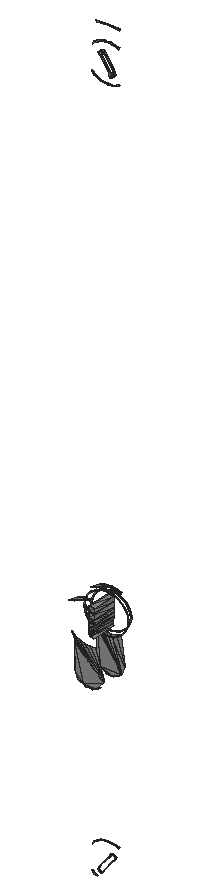
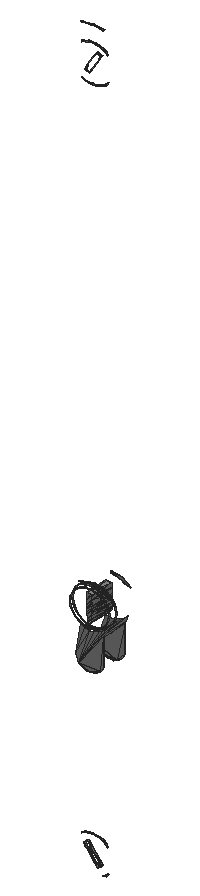
# SketchUp Ruby script. Lengths in inches.
U = 1.inch
M = Sketchup.active_model
def pt(a) = Geom::Point3d.new(a.map { |v| v * U })
def face(e, loops, mat)
  f = e.add_face(loops[0].map { |a| pt(a) })
  loops[1..].each { |l| e.add_face(l.map { |a| pt(a) }).erase! }
  f.material = f.back_material = mat if mat
  f
end
# faces: each face lists its corners as indices into pts; further lists are holes
def faces(e, pts, list, mat = nil) = list.each { |f| face(e, (f[0].is_a?(Array) ? f : [f]).map { |l| l.map { |i| pts[i] } }, mat) }
# xy, xz, yz: faces in a plane at the given z, y or x. An outline is a flat list of corners, or four numbers for a rectangle; further outlines are holes
def ring(l) = l.size == 4 ? [[l[0], l[1]], [l[2], l[1]], [l[2], l[3]], [l[0], l[3]]] : l.each_slice(2).to_a
def flat(e, list, mat, &to3) = list.each { |f| face(e, (f[0].is_a?(Array) ? f : [f]).map { |l| ring(l).map { |u, v| to3.(u, v) } }, mat) }
def xy(e, z, list, mat = nil) = flat(e, list, mat) { |x, y| [x, y, z] }
def xz(e, y, list, mat = nil) = flat(e, list, mat) { |x, z| [x, y, z] }
def yz(e, x, list, mat = nil) = flat(e, list, mat) { |y, z| [x, y, z] }
def lines(e, pts, list) = list.each { |a, b| e.add_line(pt(pts[a]), pt(pts[b])) }
# prism: a flat outline (further loops are holes) pulled along v
def prism(e, loops, v, mat = nil)
  f = face(e, loops, mat); d = Geom::Vector3d.new(v.map { |x| x * U })
  f.pushpull(f.normal.samedirection?(d) ? d.length : -d.length)
end
def box(e, o, s, mat = nil) = prism(e, [[o, [o[0] + s[0], o[1], o[2]], [o[0] + s[0], o[1] + s[1], o[2]], [o[0], o[1] + s[1], o[2]]]], [0, 0, s[2]], mat)
def at(x, y, z, deg = 0) = Geom::Transformation.translation(pt([x, y, z])) * Geom::Transformation.rotation(ORIGIN, Z_AXIS, deg.degrees)
def axes(o, x, y, z) = Geom::Transformation.new([*x, 0, *y, 0, *z, 0, *pt(o).to_a, 1])
def part(name) = M.definitions.add(name)
# library, detail: a bought-in or finely detailed component or shape, given as its bounding box
def library(name, o, s) = part(name).tap { |d| box(d.entities, o, s) }
def detail(e, o, s) = box(e.add_group.entities, o, s)
def put(e, d, t, mat = nil) = e.add_instance(d, t).tap { |i| i.material = mat if mat }
def group(e, t, mat = nil) = e.add_group.tap { |g| g.transformation = t; g.material = mat if mat }.entities
root = M.entities
M.materials.add("Material \#1").color = [140, 140, 140]
xy(root,42.551,[[1590.906,531.083,1590.906,531.406,1590.949,531.083],[1590.949,531.083,1590.906,531.406,1590.949,531.406]],"Material \#1")
xy(root,42.907,[[1590.884,531.083,1590.957,531.083,1590.957,531.406],[1590.884,531.083,1590.957,531.406,1590.884,531.406]],"Material \#1")
xz(root,531.048,[[1590.92,41.959,1590.837,41.976,1591.004,41.976],[1590.92,41.959,1590.877,41.963,1590.837,41.976],[1590.92,41.959,1591.004,41.976,1590.964,41.963],[1590.837,41.976,1590.73,42.452,1591.105,42.089],[1590.837,41.976,1590.735,42.089,1590.73,42.452],
  [1590.837,41.976,1590.772,42.022,1590.735,42.089],[1590.837,41.976,1590.801,41.996,1590.772,42.022],[1590.837,41.976,1591.105,42.089,1591.004,41.976],[1591.004,41.976,1591.068,42.022,1591.039,41.996],[1590.772,42.022,1590.749,42.054,1590.735,42.089],
  [1591.105,42.089,1590.723,42.477,1591.11,42.128],[1591.105,42.089,1590.726,42.471,1590.723,42.477],[1591.105,42.089,1590.728,42.465,1590.726,42.471],[1591.105,42.089,1590.73,42.459,1590.728,42.465],[1590.735,42.089,1590.73,42.128,1590.73,42.452],
  [1591.105,42.089,1590.73,42.452,1590.73,42.459],[1591.11,42.128,1590.686,42.562,1590.733,42.521],[1591.11,42.128,1590.723,42.477,1590.686,42.562],[1591.11,42.128,1590.733,42.521,1590.788,42.489],[1591.11,42.128,1590.788,42.489,1590.851,42.469],
  [1591.11,42.128,1590.851,42.469,1590.92,42.462],[1591.11,42.128,1590.92,42.462,1590.989,42.469],[1590.655,42.918,1590.771,43.001,1590.92,43.032],[1590.655,42.918,1590.788,42.969,1590.733,42.9375],[1590.655,42.918,1590.92,43.032,1590.788,42.969],
  [1590.788,42.969,1590.92,43.032,1590.851,42.989],[1590.851,42.989,1590.92,43.032,1590.92,42.996],[1590.771,43.001,1590.842,43.024,1590.92,43.032]],"Material \#1")
xz(root,531.083,[[1590.906,42.551,1590.935,42.578,1590.892,42.578],[1590.906,42.551,1590.949,42.551,1590.935,42.578],[1590.892,42.578,1590.943,42.587,1590.884,42.587],[1590.892,42.578,1590.935,42.578,1590.943,42.587],[1590.884,42.587,1590.943,42.587,1590.943,42.607],
  [1590.884,42.587,1590.943,42.607,1590.884,42.607],[1590.884,42.607,1590.935,42.615,1590.892,42.615],[1590.884,42.607,1590.943,42.607,1590.935,42.615],[1590.892,42.615,1590.935,42.615,1590.949,42.649],[1590.892,42.615,1590.949,42.649,1590.892,42.649],
  [1590.892,42.649,1590.949,42.649,1590.949,42.68],[1590.892,42.649,1590.949,42.68,1590.892,42.68],[1590.892,42.68,1590.96,42.705,1590.881,42.705],[1590.892,42.68,1590.949,42.68,1590.96,42.705],[1590.881,42.705,1590.96,42.705,1590.96,42.73],
  [1590.881,42.705,1590.96,42.73,1590.881,42.73],[1590.881,42.73,1590.949,42.756,1590.892,42.756],[1590.881,42.73,1590.96,42.73,1590.949,42.756],[1590.892,42.756,1590.957,42.773,1590.884,42.773],[1590.892,42.756,1590.949,42.756,1590.957,42.773],
  [1590.884,42.773,1590.957,42.773,1590.957,42.831],[1590.884,42.773,1590.957,42.831,1590.884,42.831],[1590.884,42.831,1590.948,42.836,1590.893,42.836],[1590.884,42.831,1590.957,42.831,1590.948,42.836],[1590.893,42.836,1590.948,42.836,1590.948,42.845],
  [1590.893,42.836,1590.948,42.845,1590.893,42.845],[1590.893,42.845,1590.957,42.849,1590.884,42.849],[1590.893,42.845,1590.948,42.845,1590.957,42.849],[1590.884,42.849,1590.957,42.849,1590.957,42.907],[1590.884,42.849,1590.957,42.907,1590.884,42.907]],"Material \#1")
xz(root,531.326,[[1590.92,42.462,1590.92,42.471,1590.843,42.471],[1590.92,42.462,1590.995,42.48,1590.92,42.471],[1590.92,42.462,1590.998,42.471,1590.995,42.48],[1590.843,42.471,1590.845,42.48,1590.77,42.498],[1590.843,42.471,1590.92,42.471,1590.845,42.48],
  [1590.998,42.471,1591.065,42.505,1590.995,42.48],[1590.998,42.471,1591.07,42.498,1591.065,42.505],[1590.845,42.48,1590.775,42.505,1590.77,42.498],[1590.77,42.498,1590.775,42.505,1590.708,42.54],[1591.07,42.498,1591.125,42.546,1591.065,42.505],
  [1591.07,42.498,1591.132,42.54,1591.125,42.546],[1590.775,42.505,1590.715,42.546,1590.708,42.54],[1590.708,42.54,1590.715,42.546,1590.66,42.595],[1591.132,42.54,1591.171,42.6,1591.125,42.546],[1591.132,42.54,1591.18,42.595,1591.171,42.6],
  [1590.715,42.546,1590.669,42.6,1590.66,42.595],[1590.66,42.595,1590.669,42.6,1590.63,42.66],[1591.18,42.595,1591.2,42.662,1591.171,42.6],[1591.18,42.595,1591.21,42.66,1591.2,42.662],[1590.669,42.6,1590.64,42.662,1590.63,42.66],
  [1590.63,42.66,1590.64,42.662,1590.62,42.729],[1591.21,42.66,1591.21,42.729,1591.2,42.662],[1591.21,42.66,1591.22,42.729,1591.21,42.729],[1590.64,42.662,1590.63,42.729,1590.62,42.729],[1590.62,42.729,1590.63,42.729,1590.63,42.798],
  [1590.63,42.729,1590.64,42.796,1590.63,42.798],[1591.21,42.729,1591.22,42.729,1591.2,42.796],[1591.22,42.729,1591.21,42.798,1591.2,42.796],[1590.64,42.796,1590.66,42.862,1590.63,42.798],[1590.64,42.796,1590.669,42.858,1590.66,42.862],
  [1591.2,42.796,1591.21,42.798,1591.171,42.858],[1591.21,42.798,1591.18,42.862,1591.171,42.858],[1590.669,42.858,1590.708,42.918,1590.66,42.862],[1590.669,42.858,1590.715,42.911,1590.708,42.918],[1591.171,42.858,1591.18,42.862,1591.125,42.911],
  [1591.18,42.862,1591.132,42.918,1591.125,42.911],[1590.715,42.911,1590.77,42.96,1590.708,42.918],[1590.715,42.911,1590.775,42.952,1590.77,42.96],[1591.125,42.911,1591.132,42.918,1591.065,42.952],[1591.132,42.918,1591.07,42.96,1591.065,42.952],
  [1590.775,42.952,1590.843,42.987,1590.77,42.96],[1590.775,42.952,1590.845,42.978,1590.843,42.987],[1591.065,42.952,1591.07,42.96,1590.995,42.978],[1591.07,42.96,1590.998,42.987,1590.995,42.978],[1590.845,42.978,1590.92,42.996,1590.843,42.987],
  [1590.845,42.978,1590.92,42.987,1590.92,42.996],[1590.995,42.978,1590.998,42.987,1590.92,42.987],[1590.92,42.987,1590.998,42.987,1590.92,42.996]],"Material \#1")
xz(root,531.361,[[1590.781,39.535,1590.743,39.559,1590.733,39.549],[1590.733,39.549,1590.743,39.559,1590.698,39.58],[1590.743,39.559,1590.71,39.589,1590.698,39.58],[1590.71,39.905,1590.743,39.934,1590.733,39.945],[1590.743,39.934,1590.774,39.97,1590.733,39.945],
  [1590.743,39.934,1590.781,39.959,1590.774,39.97],[1590.781,39.959,1590.819,39.989,1590.774,39.97],[1590.781,39.959,1590.824,39.977,1590.819,39.989],[1591.059,39.959,1591.067,39.97,1591.016,39.977],[1591.067,39.97,1591.021,39.989,1591.016,39.977],
  [1590.824,39.977,1590.868,40.001,1590.819,39.989],[1590.824,39.977,1590.871,39.988,1590.868,40.001],[1591.016,39.977,1591.021,39.989,1590.969,39.988],[1590.871,39.988,1590.92,40.005,1590.868,40.001],[1590.871,39.988,1590.92,39.992,1590.92,40.005],
  [1590.969,39.988,1590.972,40.001,1590.92,39.992],[1590.969,39.988,1591.021,39.989,1590.972,40.001],[1590.92,39.992,1590.972,40.001,1590.92,40.005],[1590.92,49.013,1590.92,49.027,1590.868,49.017],[1590.92,49.013,1590.969,49.031,1590.92,49.027],
  [1590.92,49.013,1590.972,49.017,1590.969,49.031],[1590.868,49.017,1590.871,49.031,1590.819,49.029],[1590.868,49.017,1590.92,49.027,1590.871,49.031],[1590.972,49.017,1591.016,49.042,1590.969,49.031],[1590.972,49.017,1591.021,49.029,1591.016,49.042],
  [1590.819,49.029,1590.824,49.042,1590.774,49.049],[1590.819,49.029,1590.871,49.031,1590.824,49.042],[1591.021,49.029,1591.059,49.06,1591.016,49.042],[1591.021,49.029,1591.067,49.049,1591.059,49.06],[1590.824,49.042,1590.781,49.06,1590.774,49.049],
  [1590.774,49.049,1590.781,49.06,1590.733,49.074],[1590.781,49.06,1590.743,49.084,1590.733,49.074],[1590.733,49.074,1590.743,49.084,1590.698,49.105],[1590.743,49.084,1590.71,49.114,1590.698,49.105],[1590.71,49.43,1590.743,49.459,1590.733,49.47],
  [1590.743,49.459,1590.774,49.495,1590.733,49.47],[1590.743,49.459,1590.781,49.484,1590.774,49.495],[1590.781,49.484,1590.819,49.514,1590.774,49.495],[1590.781,49.484,1590.824,49.502,1590.819,49.514],[1591.059,49.484,1591.067,49.495,1591.016,49.502],
  [1591.067,49.495,1591.021,49.514,1591.016,49.502],[1590.824,49.502,1590.868,49.526,1590.819,49.514],[1590.824,49.502,1590.871,49.513,1590.868,49.526],[1591.016,49.502,1591.021,49.514,1590.969,49.513],[1590.871,49.513,1590.92,49.53,1590.868,49.526],
  [1590.871,49.513,1590.92,49.517,1590.92,49.53],[1590.969,49.513,1590.972,49.526,1590.92,49.517],[1590.969,49.513,1591.021,49.514,1590.972,49.526],[1590.92,49.517,1590.972,49.526,1590.92,49.53],[1590.766,49.713,1590.92,49.739,1590.763,49.726],
  [1590.766,49.713,1590.92,49.725,1590.92,49.739],[1591.075,49.713,1591.077,49.726,1590.92,49.725],[1590.92,49.725,1591.077,49.726,1590.92,49.739]],"Material \#1")
xz(root,531.396,[[1590.92,41.959,1590.772,42.022,1590.837,41.976],[1590.92,41.959,1591.068,42.022,1590.772,42.022],[1590.92,41.959,1590.837,41.976,1590.877,41.963],[1590.92,41.959,1590.964,41.963,1591.004,41.976],[1590.92,41.959,1591.004,41.976,1591.068,42.022],
  [1590.837,41.976,1590.772,42.022,1590.801,41.996],[1591.004,41.976,1591.039,41.996,1591.068,42.022],[1591.068,42.022,1590.583,42.689,1590.723,42.477],[1591.068,42.022,1590.686,42.562,1590.583,42.689],[1591.068,42.022,1590.733,42.521,1590.686,42.562],
  [1591.068,42.022,1590.723,42.477,1590.726,42.471],[1591.068,42.022,1590.726,42.471,1590.728,42.465],[1591.068,42.022,1590.728,42.465,1590.73,42.459],[1590.772,42.022,1590.73,42.452,1590.735,42.089],[1590.772,42.022,1590.73,42.459,1590.73,42.452],
  [1590.772,42.022,1591.068,42.022,1590.73,42.459],[1591.068,42.022,1590.788,42.489,1590.733,42.521],[1590.772,42.022,1590.735,42.089,1590.75,42.054],[1591.068,42.022,1590.851,42.469,1590.788,42.489],[1591.068,42.022,1590.92,42.462,1590.851,42.469],
  [1591.068,42.022,1591.11,42.128,1590.92,42.462],[1590.735,42.089,1590.73,42.452,1590.73,42.128],[1591.11,42.128,1590.989,42.469,1590.92,42.462],[1591.11,42.128,1591.052,42.489,1590.989,42.469],[1590.655,42.918,1590.733,42.9375,1590.788,42.969],
  [1590.655,42.918,1590.788,42.969,1590.92,43.032],[1590.655,42.918,1590.92,43.032,1590.771,43.001],[1590.788,42.969,1590.851,42.989,1590.92,43.032],[1591.052,42.969,1590.92,43.032,1590.989,42.989],[1590.851,42.989,1590.92,42.996,1590.92,43.032],
  [1590.989,42.989,1590.92,43.032,1590.92,42.996],[1590.771,43.001,1590.92,43.032,1590.842,43.024],[1591.07,43.001,1590.998,43.024,1590.92,43.032]],"Material \#1")
xz(root,531.406,[[1590.92,42.491,1590.92,42.5,1590.851,42.499],[1590.92,42.491,1590.987,42.508,1590.92,42.5],[1590.92,42.491,1590.989,42.499,1590.987,42.508],[1590.851,42.499,1590.854,42.508,1590.786,42.523],[1590.851,42.499,1590.92,42.5,1590.854,42.508],
  [1590.989,42.499,1591.049,42.531,1590.987,42.508],[1590.989,42.499,1591.054,42.523,1591.049,42.531],[1590.854,42.508,1590.792,42.531,1590.786,42.523],[1590.786,42.523,1590.792,42.531,1590.731,42.561],[1591.054,42.523,1591.102,42.567,1591.049,42.531],
  [1591.054,42.523,1591.109,42.561,1591.102,42.567],[1590.792,42.531,1590.738,42.567,1590.731,42.561],[1590.731,42.561,1590.738,42.567,1590.689,42.61],[1591.109,42.561,1591.143,42.614,1591.102,42.567],[1591.109,42.561,1591.152,42.61,1591.143,42.614],
  [1590.738,42.567,1590.697,42.614,1590.689,42.61],[1590.689,42.61,1590.697,42.614,1590.662,42.667],[1591.152,42.61,1591.169,42.67,1591.143,42.614],[1591.152,42.61,1591.178,42.667,1591.169,42.67],[1590.697,42.614,1590.672,42.67,1590.662,42.667],
  [1590.662,42.667,1590.672,42.67,1590.653,42.729],[1591.178,42.667,1591.177,42.729,1591.169,42.67],[1591.178,42.667,1591.1875,42.729,1591.177,42.729],[1590.672,42.67,1590.663,42.729,1590.653,42.729],[1590.653,42.729,1590.663,42.729,1590.662,42.791],
  [1590.663,42.729,1590.672,42.788,1590.662,42.791],[1591.177,42.729,1591.1875,42.729,1591.169,42.788],[1591.1875,42.729,1591.178,42.791,1591.169,42.788],[1590.672,42.788,1590.689,42.848,1590.662,42.791],[1590.672,42.788,1590.697,42.843,1590.689,42.848],
  [1591.169,42.788,1591.178,42.791,1591.143,42.843],[1591.178,42.791,1591.152,42.848,1591.143,42.843],[1590.697,42.843,1590.731,42.897,1590.689,42.848],[1590.697,42.843,1590.738,42.891,1590.731,42.897],[1591.143,42.843,1591.152,42.848,1591.102,42.891],
  [1591.152,42.848,1591.109,42.897,1591.102,42.891],[1590.738,42.891,1590.786,42.935,1590.731,42.897],[1590.738,42.891,1590.792,42.927,1590.786,42.935],[1591.102,42.891,1591.109,42.897,1591.049,42.927],[1591.109,42.897,1591.054,42.935,1591.049,42.927],
  [1590.792,42.927,1590.851,42.959,1590.786,42.935],[1590.792,42.927,1590.854,42.95,1590.851,42.959],[1591.049,42.927,1591.054,42.935,1590.987,42.95],[1591.054,42.935,1590.989,42.959,1590.987,42.95],[1590.854,42.95,1590.92,42.967,1590.851,42.959],
  [1590.854,42.95,1590.92,42.958,1590.92,42.967],[1590.987,42.95,1590.989,42.959,1590.92,42.958],[1590.92,42.958,1590.989,42.959,1590.92,42.967]],"Material \#1")
yz(root,1590.884,[[531.083,42.849,531.083,42.907,531.406,42.907]],"Material \#1")
yz(root,1590.892,[[531.083,42.615,531.083,42.649,531.406,42.649]],"Material \#1")
yz(root,1590.949,[[531.083,42.649,531.406,42.649,531.083,42.68],[531.406,42.649,531.406,42.68,531.083,42.68]],"Material \#1")
yz(root,1590.957,[[531.083,42.773,531.406,42.773,531.083,42.831]],"Material \#1")
yz(root,1590.96,[[531.083,42.705,531.406,42.705,531.083,42.73],[531.406,42.705,531.406,42.73,531.083,42.73]],"Material \#1")
p = [[1590.82,531.361,39.672],[1590.798,531.354,39.644],[1590.798,531.326,39.644],[1590.82,531.334,39.672],[1590.823,531.354,39.623],[1590.823,531.326,39.623],
  [1590.854,531.354,39.609],[1590.854,531.326,39.609],[1590.875,531.361,39.637],[1590.875,531.334,39.637],[1590.895,531.364,39.662],[1590.895,531.336,39.662],
  [1590.945,531.364,39.831],[1590.84,531.364,39.697],[1590.84,531.336,39.697],[1590.945,531.336,39.831],[1591.001,531.364,39.797],[1591.001,531.336,39.797],
  [1590.965,531.361,39.856],[1590.965,531.334,39.856],[1591.02,531.361,39.822],[1591.02,531.334,39.822],[1591.043,531.354,39.849],[1591.043,531.326,39.849],
  [1591.017,531.354,39.87],[1591.017,531.326,39.87],[1590.987,531.354,39.884],[1590.987,531.326,39.884],[1590.888,531.406,42.582],[1590.906,531.406,42.551],
  [1590.906,531.083,42.551],[1590.892,531.083,42.578],[1590.888,531.406,42.582],[1590.949,531.083,42.649],[1590.935,531.083,42.615],[1590.939,531.406,42.611],
  [1590.939,531.406,42.611],[1590.935,531.083,42.615],[1590.943,531.083,42.607],[1590.939,531.406,42.582],[1590.943,531.083,42.587],[1590.935,531.083,42.578],
  [1590.935,531.083,42.578],[1590.949,531.083,42.551],[1590.949,531.406,42.551],[1590.888,531.406,42.611],[1590.884,531.083,42.607],[1590.892,531.083,42.615],
  [1590.888,531.406,42.582],[1590.892,531.083,42.578],[1590.884,531.083,42.587],[1590.892,531.083,42.649],[1590.892,531.083,42.68],[1590.886,531.406,42.693],
  [1590.939,531.406,42.582],[1590.939,531.406,42.611],[1590.943,531.083,42.607],[1590.943,531.083,42.587],[1590.888,531.406,42.611],[1590.888,531.406,42.582],
  [1590.884,531.083,42.587],[1590.884,531.083,42.607],[1590.939,531.406,42.611],[1590.949,531.406,42.649],[1590.949,531.083,42.649],[1590.949,531.406,42.551],
  [1590.939,531.406,42.582],[1590.935,531.083,42.578],[1590.892,531.406,42.649],[1590.888,531.406,42.611],[1590.892,531.083,42.615],[1590.886,531.406,42.693],
  [1590.892,531.406,42.649],[1590.892,531.083,42.649],[1590.949,531.083,42.756],[1590.96,531.083,42.73],[1590.96,531.406,42.73],[1590.881,531.083,42.73],
  [1590.892,531.083,42.756],[1590.888,531.406,42.765],[1590.881,531.083,42.705],[1590.881,531.083,42.73],[1590.886,531.406,42.743],[1590.892,531.083,42.68],
  [1590.881,531.083,42.705],[1590.881,531.406,42.718],[1590.949,531.406,42.68],[1590.96,531.406,42.705],[1590.96,531.083,42.705],[1590.949,531.083,42.68],
  [1590.96,531.406,42.73],[1590.949,531.406,42.756],[1590.949,531.083,42.756],[1590.888,531.406,42.765],[1590.886,531.406,42.743],[1590.881,531.083,42.73],
  [1590.886,531.406,42.743],[1590.881,531.406,42.718],[1590.881,531.083,42.705],[1590.881,531.406,42.718],[1590.886,531.406,42.693],[1590.892,531.083,42.68],
  [1590.953,531.406,42.842],[1590.948,531.083,42.836],[1590.957,531.083,42.831],[1590.888,531.406,42.836],[1590.893,531.083,42.836],[1590.893,531.083,42.845],
  [1590.888,531.406,42.836],[1590.884,531.083,42.849],[1590.888,531.406,42.836],[1590.884,531.083,42.831],[1590.953,531.406,42.842],[1590.957,531.083,42.849],
  [1590.948,531.083,42.845],[1590.953,531.406,42.842],[1590.957,531.083,42.773],[1590.949,531.083,42.756],[1590.949,531.406,42.756],[1590.884,531.083,42.773],
  [1590.884,531.083,42.831],[1590.888,531.406,42.836],[1590.892,531.083,42.756],[1590.884,531.083,42.773],[1590.885,531.406,42.777],[1590.949,531.406,42.756],
  [1590.957,531.406,42.773],[1590.957,531.083,42.773],[1590.884,531.406,42.907],[1590.888,531.406,42.836],[1590.884,531.083,42.849],[1590.888,531.406,42.836],
  [1590.885,531.406,42.777],[1590.884,531.083,42.773],[1590.885,531.406,42.777],[1590.888,531.406,42.765],[1590.892,531.083,42.756],[1590.957,531.083,42.907],
  [1590.957,531.083,42.849],[1590.953,531.406,42.842],[1590.953,531.406,42.842],[1590.957,531.406,42.907],[1590.957,531.083,42.907],[1590.957,531.406,42.773],
  [1590.953,531.406,42.842],[1590.957,531.083,42.831],[1590.954,531.361,49.159],[1590.973,531.354,49.13],[1590.973,531.326,49.13],[1590.954,531.334,49.159],
  [1591.005,531.354,49.141],[1591.005,531.326,49.141],[1591.032,531.354,49.16],[1591.032,531.326,49.16],[1590.845,531.364,49.328],[1590.937,531.364,49.186],
  [1590.937,531.336,49.186],[1590.845,531.336,49.328],[1590.996,531.364,49.216],[1590.903,531.364,49.358],[1590.903,531.336,49.358],[1590.996,531.336,49.216],
  [1591.013,531.361,49.189],[1591.013,531.334,49.189],[1590.828,531.361,49.354],[1590.828,531.334,49.354],[1590.867,531.354,49.414],[1590.836,531.354,49.402],
  [1590.836,531.326,49.402],[1590.867,531.326,49.414],[1590.809,531.354,49.384],[1590.809,531.326,49.384],[1590.886,531.361,49.384],[1590.886,531.334,49.384]]
faces(root,p,[[0,1,2],[2,3,0],[1,4,5],[5,2,1],[4,6,7],[7,5,4],[6,8,9],[9,7,6],
  [8,10,11],[11,9,8],[12,13,14],[14,15,12],[13,0,3],[3,14,13],[10,16,17],[17,11,10],
  [18,12,15],[15,19,18],[16,20,21],[21,17,16],[20,22,23],[23,21,20],[22,24,25],[25,23,22],
  [24,26,27],[27,25,24],[26,18,19],[19,27,26],[28,29,30],[30,31,32],[33,34,35],[36,37,38],
  [39,40,41],[42,43,44],[45,46,47],[48,49,50],[51,52,53],[54,55,56],[56,57,54],[58,59,60],
  [60,61,58],[62,63,64],[65,66,67],[68,69,70],[71,72,73],[74,75,76],[77,78,79],[80,81,82],
  [83,84,85],[86,87,88],[88,89,86],[90,91,92],[93,94,95],[96,97,98],[99,100,101],[102,103,104],
  [105,106,107],[108,107,109],[110,111,106],[112,113,114],[115,114,103],[116,117,118],[119,120,121],[122,123,124],
  [125,126,127],[128,129,130],[131,132,133],[134,135,136],[137,138,139],[140,141,142],[143,144,145],[146,147,148],
  [148,149,146],[147,150,151],[151,148,147],[150,152,153],[153,151,150],[154,155,156],[156,157,154],[155,146,149],
  [149,156,155],[158,159,160],[160,161,158],[152,162,163],[163,153,152],[162,158,161],[161,163,162],[164,154,157],
  [157,165,164],[166,167,168],[168,169,166],[167,170,171],[171,168,167],[170,164,165],[165,171,170],[159,172,173],
  [173,160,159],[172,166,169],[169,173,172]],"Material \#1")
